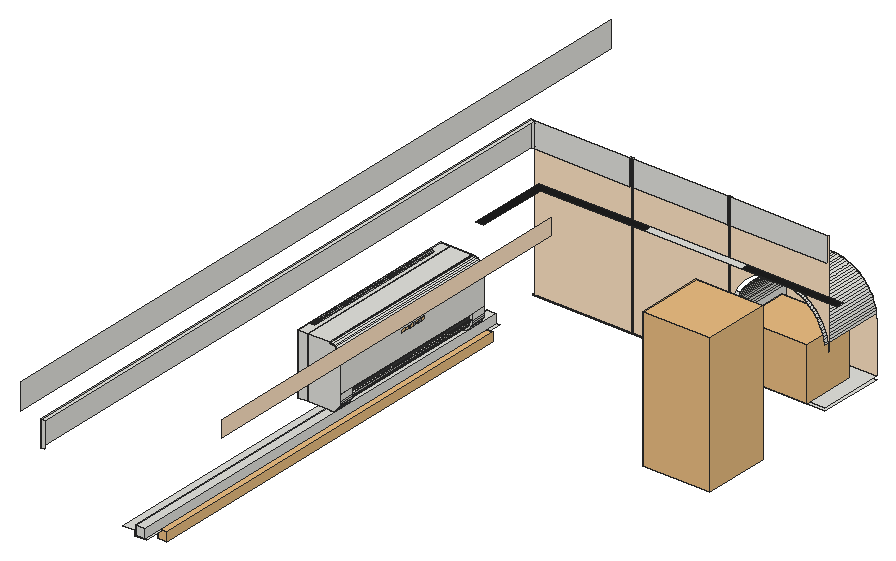
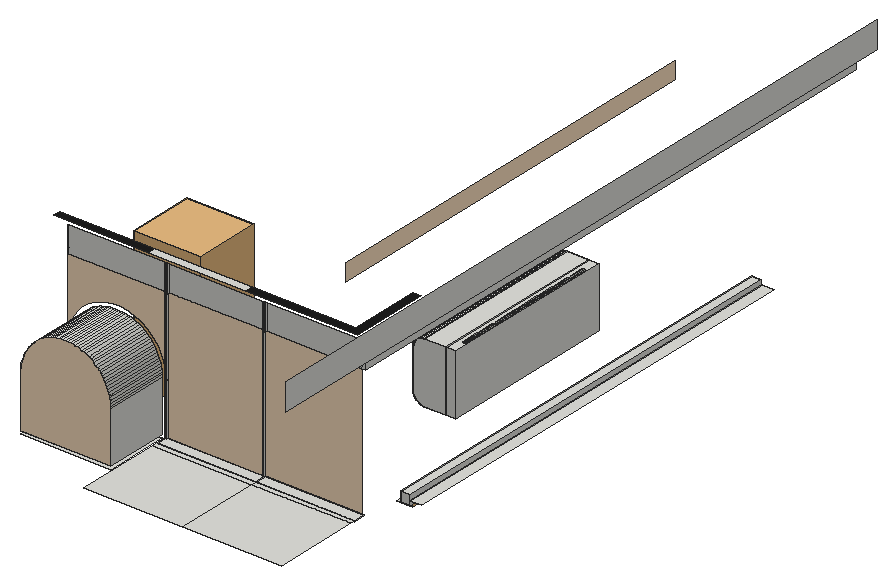
# SketchUp Ruby script. Lengths in inches.
U = 1.inch
M = Sketchup.active_model
def pt(a) = Geom::Point3d.new(a.map { |v| v * U })
def face(e, loops, mat)
  f = e.add_face(loops[0].map { |a| pt(a) })
  loops[1..].each { |l| e.add_face(l.map { |a| pt(a) }).erase! }
  f.material = f.back_material = mat if mat
  f
end
# faces: each face lists its corners as indices into pts; further lists are holes
def faces(e, pts, list, mat = nil) = list.each { |f| face(e, (f[0].is_a?(Array) ? f : [f]).map { |l| l.map { |i| pts[i] } }, mat) }
# xy, xz, yz: faces in a plane at the given z, y or x. An outline is a flat list of corners, or four numbers for a rectangle; further outlines are holes
def ring(l) = l.size == 4 ? [[l[0], l[1]], [l[2], l[1]], [l[2], l[3]], [l[0], l[3]]] : l.each_slice(2).to_a
def flat(e, list, mat, &to3) = list.each { |f| face(e, (f[0].is_a?(Array) ? f : [f]).map { |l| ring(l).map { |u, v| to3.(u, v) } }, mat) }
def xy(e, z, list, mat = nil) = flat(e, list, mat) { |x, y| [x, y, z] }
def xz(e, y, list, mat = nil) = flat(e, list, mat) { |x, z| [x, y, z] }
def yz(e, x, list, mat = nil) = flat(e, list, mat) { |y, z| [x, y, z] }
def lines(e, pts, list) = list.each { |a, b| e.add_line(pt(pts[a]), pt(pts[b])) }
# prism: a flat outline (further loops are holes) pulled along v
def prism(e, loops, v, mat = nil)
  f = face(e, loops, mat); d = Geom::Vector3d.new(v.map { |x| x * U })
  f.pushpull(f.normal.samedirection?(d) ? d.length : -d.length)
end
def box(e, o, s, mat = nil) = prism(e, [[o, [o[0] + s[0], o[1], o[2]], [o[0] + s[0], o[1] + s[1], o[2]], [o[0], o[1] + s[1], o[2]]]], [0, 0, s[2]], mat)
def at(x, y, z, deg = 0) = Geom::Transformation.translation(pt([x, y, z])) * Geom::Transformation.rotation(ORIGIN, Z_AXIS, deg.degrees)
def axes(o, x, y, z) = Geom::Transformation.new([*x, 0, *y, 0, *z, 0, *pt(o).to_a, 1])
def part(name) = M.definitions.add(name)
# library, detail: a bought-in or finely detailed component or shape, given as its bounding box
def library(name, o, s) = part(name).tap { |d| box(d.entities, o, s) }
def detail(e, o, s) = box(e.add_group.entities, o, s)
def put(e, d, t, mat = nil) = e.add_instance(d, t).tap { |i| i.material = mat if mat }
def group(e, t, mat = nil) = e.add_group.tap { |g| g.transformation = t; g.material = mat if mat }.entities
root = M.entities
M.materials.add("[0012_Bisque]").color = [255, 228, 196]
M.materials.add("[Color M08]").color = [30, 30, 30]
M.materials.add("[Color_004]").color = [142, 142, 142]
M.materials.add("[Color_007]").color = [58, 58, 58]
M.materials.add("[Color_C12]").color = [153, 91, 30]
c1 = library("Curtain rod",[-0.76,-0.76,-71.54],[3.88,3.88,152.54])
c2 = library("Group\#26",[-80.34,-149.03,-93.91],[1.18,2.79,3])
c3 = library("Group\#27",[-80.34,-139.83,-93.89],[1.18,2.84,2.98])
c4 = library("Group\#19",[-80.46,-65.36,-92.6],[1.38,3.58,3.59])
c5 = library("Group\#15",[-88.79,0.67,-41.3125],[0.99,6.14,4.87])
c6 = library("Group\#18",[-88.79,21.34,-41.3125],[0.99,6.53,4.87])
c7 = library("books",[6.19,-1.3125,-0.22],[15.35,11.9,12.07])
c8 = library("Group\#46",[0,0,0],[110.16,110.16,227.25])
xy(root,87,[[[2.71,29.49,5.62,131.05],[2.85,29.63,4.97,130.91]]])
xy(root,88.0625,[[0,29.49,2.71,131.05]])
xy(root,88.24,[[51.69,141.2,72.61,155.95]])
xy(root,88.4375,[[5.12,141.2,5.62,143.84],[5.62,141.2,27.93,143.84],[27.93,141.2,50.74,143.84],[27.56,143.84,27.93,144.02]])
xy(root,88.6875,[[5.12,141.2,27.93,143.84],[27.93,141.2,28.23,141.5],[28.23,141.2,50.44,141.2,50.44,141.5,50.74,141.5,50.74,143.84,27.93,143.84,27.93,141.5,28.23,141.5],[50.44,141.2,50.74,141.5],[5.12,143.84,27.93,145.09],
  [27.93,143.84,50.74,145.09],[5.12,145.09,27.93,164.88],[27.93,145.09,50.74,164.88]])
xy(root,88.95,[[51.69,141.2,72.61,155.95]])
xy(root,89.125,[[2.85,29.63,4.97,130.91]])
xy(root,118.75,[[39.875,130.07,62.26,131.88]])
xy(root,118.75,[[14.13,113.7,14.13,131.88,39.875,131.88,39.875,130.07,15.9375,130.07,15.9375,113.7],[62.26,130.07,84.16,131.88]],"[Color M08]")
xy(root,124.6875,[[4.82,0,5.62,141.2],[27.63,141.2,27.93,141.5],[27.93,141.2,28.23,141.5],[50.14,141.2,50.44,141.5],[50.44,141.2,50.74,141.5]])
xz(root,0,[[4.82,118.75,5.62,124.6875]])
xz(root,29.63,[[2.85,87,4.97,89.125]])
xz(root,130.91,[[2.85,87,4.97,89.125]])
xz(root,141.2,[[5.12,88.4375,5.62,88.6875],[5.62,88.4375,27.93,88.6875],[27.93,88.4375,50.74,88.6875],[4.82,118.75,5.62,124.6875],[5.62,118.75,27.63,124.6875],
  [27.93,118.75,28.23,124.6875],[28.23,118.75,50.14,124.6875],[50.44,118.75,50.74,124.6875],[50.74,118.75,73.26,124.6875]])
xz(root,141.2,[[5.62,88.6875,27.93,88.6875,27.93,124.6875,27.63,124.6875,27.63,118.75,5.62,118.75],[28.23,88.6875,50.44,88.6875,50.44,124.6875,50.14,124.6875,50.14,118.75,28.23,118.75],[50.74,100.6875,50.76,101.28,50.81,101.88,50.88,102.47,50.99,103.06,51.13,103.64,51.3,104.21,51.5,104.78,51.73,105.33,51.99,105.87,52.27,106.39,52.58,106.9,52.92,107.39,53.29,107.87,53.67,108.32,54.09,108.75,54.52,109.16,54.97,109.55,55.45,109.92,55.9375,110.25,56.45,110.57,56.97,110.85,57.51,111.11,58.0625,111.34,58.625,111.54,59.2,111.71,59.78,111.85,60.37,111.95,60.96,112.03,61.55,112.08,62.15,112.09,62.75,112.08,63.34,112.03,63.9375,111.95,64.52,111.85,65.1,111.71,65.68,111.54,66.24,111.34,66.79,111.11,67.33,110.85,67.85,110.57,68.36,110.25,68.86,109.92,69.33,109.55,69.78,109.16,70.22,108.75,70.63,108.32,71.02,107.87,71.38,107.39,71.72,106.9,72.03,106.39,72.32,105.87,72.57,105.33,72.8,104.78,73,104.21,73.17,103.64,73.31,103.06,73.42,102.47,73.5,101.88,73.54,101.28,73.56,100.6875,73.56,124.6875,73.26,124.6875,73.26,118.75,50.74,118.75]],"[0012_Bisque]")
xz(root,141.5,[[27.93,88.6875,28.23,124.6875],[50.44,88.6875,50.74,124.6875],[27.63,118.75,27.93,124.6875],[50.14,118.75,50.44,124.6875]])
xz(root,143.84,[[5.12,88.4375,27.93,88.6875],[27.93,88.4375,50.74,88.6875]])
xz(root,155.95,[[51.69,88.95,72.61,88.95,72.61,100.6875,72.59,101.23,72.55,101.78,72.48,102.32,72.38,102.86,72.25,103.39,72.1,103.92,71.91,104.43,71.7,104.94,71.47,105.43,71.21,105.92,70.92,106.38,70.61,106.83,70.28,107.27,69.92,107.68,69.55,108.08,69.15,108.46,68.73,108.8125,68.3,109.15,67.85,109.46,67.38,109.74,66.9,110,66.4,110.24,65.9,110.45,65.38,110.63,64.86,110.79,64.33,110.92,63.79,111.02,63.24,111.09,62.7,111.13,62.15,111.14,61.6,111.13,61.06,111.09,60.52,111.02,59.98,110.92,59.44,110.79,58.92,110.63,58.4,110.45,57.9,110.24,57.4,110,56.92,109.74,56.46,109.46,56,109.15,55.57,108.8125,55.15,108.46,54.76,108.08,54.38,107.68,54.02,107.27,53.69,106.83,53.38,106.38,53.1,105.92,52.83,105.43,52.6,104.94,52.39,104.43,52.21,103.92,52.05,103.39,51.92,102.86,51.82,102.32,51.75,101.78,51.71,101.23,51.69,100.6875]],"[0012_Bisque]")
yz(root,0,[[0,124.6875,170.3125,130.6875]])
yz(root,2.71,[[29.49,87,131.05,88.0625]])
yz(root,2.85,[[29.63,87,130.91,89.125]])
yz(root,4.82,[[0,118.75,141.2,124.6875]])
yz(root,4.97,[[29.63,87,130.91,89.125]])
yz(root,5.12,[[141.2,88.4375,143.84,88.6875]])
yz(root,27.63,[[141.2,118.75,141.5,124.6875]])
yz(root,27.93,[[141.2,88.4375,143.84,88.6875],[141.2,88.6875,141.5,118.75],[141.2,118.75,141.5,124.6875]])
yz(root,27.94,[[23.13,118.75,118.07,122.5625]],"[0012_Bisque]")
yz(root,28.23,[[141.2,88.6875,141.5,124.6875]])
yz(root,50.14,[[141.2,118.75,141.5,124.6875]])
yz(root,50.44,[[141.2,88.6875,141.5,100.6875],[141.2,100.6875,141.5,118.75],[141.2,118.75,141.5,124.6875]])
yz(root,50.74,[[141.2,88.4375,143.84,88.6875],[141.2,88.6875,141.5,100.6875],[141.2,100.6875,141.5,124.6875]])
yz(root,51.69,[[141.2,88.95,155.95,100.6875]])
p = [[51.71,141.2,101.23],[51.69,141.2,100.6875],[51.69,155.95,100.6875],[51.71,155.95,101.23],[51.75,141.2,101.78],[51.75,155.95,101.78],
  [51.82,141.2,102.32],[51.82,155.95,102.32],[72.55,141.2,101.78],[72.48,141.2,102.32],[72.48,155.95,102.32],[72.55,155.95,101.78],
  [51.92,141.2,102.86],[51.92,155.95,102.86],[72.38,141.2,102.86],[72.38,155.95,102.86],[52.05,141.2,103.39],[52.05,155.95,103.39],
  [72.25,141.2,103.39],[72.25,155.95,103.39],[52.21,141.2,103.92],[52.21,155.95,103.92],[72.1,141.2,103.92],[72.1,155.95,103.92],
  [52.39,141.2,104.43],[52.39,155.95,104.43],[71.91,141.2,104.43],[71.91,155.95,104.43],[52.6,141.2,104.94],[52.6,155.95,104.94],
  [71.7,141.2,104.94],[71.7,155.95,104.94],[52.83,141.2,105.43],[52.83,155.95,105.43],[71.47,141.2,105.43],[71.47,155.95,105.43],
  [53.1,141.2,105.92],[53.1,155.95,105.92],[71.21,141.2,105.92],[71.21,155.95,105.92],[53.38,141.2,106.38],[53.38,155.95,106.38],
  [70.92,141.2,106.38],[70.92,155.95,106.38],[53.69,141.2,106.83],[53.69,155.95,106.83],[70.61,141.2,106.83],[70.61,155.95,106.83],
  [54.02,141.2,107.27],[54.02,155.95,107.27],[70.28,141.2,107.27],[70.28,155.95,107.27],[54.38,141.2,107.68],[54.38,155.95,107.68],
  [69.92,141.2,107.68],[69.92,155.95,107.68],[54.76,141.2,108.08],[54.76,155.95,108.08],[69.55,141.2,108.08],[69.55,155.95,108.08],
  [55.15,141.2,108.46],[55.15,155.95,108.46],[69.15,141.2,108.46],[69.15,155.95,108.46],[55.57,141.2,108.8125],[55.57,155.95,108.8125],
  [68.73,141.2,108.8125],[68.73,155.95,108.8125],[56,141.2,109.15],[56,155.95,109.15],[68.3,141.2,109.15],[68.3,155.95,109.15],
  [56.46,141.2,109.46],[56.46,155.95,109.46],[67.85,141.2,109.46],[67.85,155.95,109.46],[56.92,141.2,109.74],[56.92,155.95,109.74],
  [67.38,141.2,109.74],[67.38,155.95,109.74],[57.4,141.2,110],[57.4,155.95,110],[66.9,141.2,110],[66.9,155.95,110],
  [57.9,141.2,110.24],[57.9,155.95,110.24],[66.4,141.2,110.24],[66.4,155.95,110.24],[58.4,141.2,110.45],[58.4,155.95,110.45],
  [65.9,141.2,110.45],[65.9,155.95,110.45],[58.92,141.2,110.63],[58.92,155.95,110.63],[65.38,141.2,110.63],[65.38,155.95,110.63],
  [59.44,141.2,110.79],[59.44,155.95,110.79],[64.86,141.2,110.79],[64.86,155.95,110.79],[59.98,141.2,110.92],[59.98,155.95,110.92],
  [64.33,141.2,110.92],[64.33,155.95,110.92],[60.52,141.2,111.02],[60.52,155.95,111.02],[63.79,141.2,111.02],[63.79,155.95,111.02],
  [61.06,141.2,111.09],[61.06,155.95,111.09],[63.24,141.2,111.09],[63.24,155.95,111.09],[61.6,141.2,111.13],[61.6,155.95,111.13],
  [62.15,141.2,111.14],[62.15,155.95,111.14],[62.7,141.2,111.13],[62.7,155.95,111.13]]
faces(root,p,[[0,1,2,3],[4,0,3,5],[6,4,5,7],[8,9,10,11],[12,6,7,13],[9,14,15,10],[16,12,13,17],[14,18,19,15],
  [20,16,17,21],[18,22,23,19],[24,20,21,25],[22,26,27,23],[28,24,25,29],[26,30,31,27],[32,28,29,33],[30,34,35,31],
  [36,32,33,37],[34,38,39,35],[40,36,37,41],[38,42,43,39],[44,40,41,45],[42,46,47,43],[48,44,45,49],[46,50,51,47],
  [52,48,49,53],[50,54,55,51],[56,52,53,57],[54,58,59,55],[60,56,57,61],[58,62,63,59],[64,60,61,65],[62,66,67,63],
  [68,64,65,69],[66,70,71,67],[72,68,69,73],[70,74,75,71],[76,72,73,77],[74,78,79,75],[80,76,77,81],[78,82,83,79],
  [84,80,81,85],[82,86,87,83],[88,84,85,89],[86,90,91,87],[92,88,89,93],[90,94,95,91],[96,92,93,97],[94,98,99,95],
  [100,96,97,101],[98,102,103,99],[104,100,101,105],[102,106,107,103],[108,104,105,109],[106,110,111,107],[112,108,109,113],[114,112,113,115],
  [116,114,115,117],[110,116,117,111]])
put(root,c1,axes([4.76,78.21,86.66],[0,0,-0.55078],[0.55078,0,0],[0,0.61526,0]))
g1 = group(root,at(5.12,94.18,110.96))
xy(g1,-13.99,[[0,-20.6,2.23,20.6]])
xy(g1,-2.49,[[0.18,-17.22,0.45,-13.11],[0.5625,-17.22,0.83,-13.11],[0.9375,-17.22,1.21,-13.11],[0.18,-12.88,0.45,-8.77],[0.5625,-12.88,0.83,-8.77],
  [0.9375,-12.88,1.21,-8.77],[0.18,-8.55,0.45,-4.44],[0.5625,-8.55,0.83,-4.44],[0.9375,-8.55,1.21,-4.44],[0.18,-4.22,0.45,-0.11],
  [0.5625,-4.22,0.83,-0.11],[0.9375,-4.22,1.21,-0.11],[0.18,0.11,0.45,4.22],[0.5625,0.11,0.83,4.22],[0.9375,0.11,1.21,4.22],
  [0.18,4.44,0.45,8.55],[0.5625,4.44,0.83,8.55],[0.9375,4.44,1.21,8.55],[0.18,8.77,0.45,12.88],[0.5625,8.77,0.83,12.88],
  [0.9375,8.77,1.21,12.88],[0.18,13.11,0.45,17.22],[0.5625,13.11,0.83,17.22],[0.9375,13.11,1.21,17.22]])
xy(g1,0,[[[0,-20.6,2.23,20.6],[0.9375,-12.88,0.9375,-8.77,1.21,-8.77,1.21,-8.55,0.9375,-8.55,0.9375,-4.44,1.21,-4.44,1.21,-12.88],[0.18,-12.88,0.18,-4.44,0.45,-4.44,0.45,-8.55,0.18,-8.55,0.18,-8.77,0.45,-8.77,0.45,-12.88],[0.5625,-17.22,0.83,-13.11],[0.18,-17.22,0.45,-13.11],[0.9375,-17.22,1.21,-13.11],[0.9375,13.11,1.21,17.22],[0.18,13.11,0.45,17.22],[0.5625,13.11,0.83,17.22],[0.5625,-8.55,0.83,-4.44],[0.18,4.44,0.45,8.55],[0.5625,4.44,0.83,8.55],[0.9375,4.44,1.21,8.55],[0.5625,-12.88,0.83,-8.77],[0.5625,-4.22,0.83,-0.11],[0.18,-4.22,0.45,-0.11],[0.9375,-4.22,1.21,-0.11],[0.18,8.77,0.45,12.88],[0.9375,8.77,1.21,12.88],[0.9375,0.11,1.21,4.22],[0.5625,0.11,0.83,4.22],[0.18,0.11,0.45,4.22],[0.5625,8.77,0.83,12.88]]])
xz(g1,-20.6,[[0,-13.99,2.23,0]])
xz(g1,-17.22,[[0.18,-2.49,0.45,0],[0.5625,-2.49,0.83,0],[0.9375,-2.49,1.21,0]])
xz(g1,-13.11,[[0.18,-2.49,0.45,0],[0.5625,-2.49,0.83,0],[0.9375,-2.49,1.21,0]])
xz(g1,-12.88,[[0.18,-2.49,0.45,0],[0.5625,-2.49,0.83,0],[0.9375,-2.49,1.21,0]])
xz(g1,-8.77,[[0.18,-2.49,0.45,0],[0.5625,-2.49,0.83,0],[0.9375,-2.49,1.21,0]])
xz(g1,-8.55,[[0.18,-2.49,0.45,0],[0.5625,-2.49,0.83,0],[0.9375,-2.49,1.21,0]])
xz(g1,-4.44,[[0.18,-2.49,0.45,0],[0.5625,-2.49,0.83,0],[0.9375,-2.49,1.21,0]])
xz(g1,-4.22,[[0.18,-2.49,0.45,0],[0.5625,-2.49,0.83,0],[0.9375,-2.49,1.21,0]])
xz(g1,-0.11,[[0.18,-2.49,0.45,0],[0.5625,-2.49,0.83,0],[0.9375,-2.49,1.21,0]])
xz(g1,0.11,[[0.18,-2.49,0.45,0],[0.5625,-2.49,0.83,0],[0.9375,-2.49,1.21,0]])
xz(g1,4.22,[[0.18,-2.49,0.45,0],[0.5625,-2.49,0.83,0],[0.9375,-2.49,1.21,0]])
xz(g1,4.44,[[0.18,-2.49,0.45,0],[0.5625,-2.49,0.83,0],[0.9375,-2.49,1.21,0]])
xz(g1,8.55,[[0.18,-2.49,0.45,0],[0.5625,-2.49,0.83,0],[0.9375,-2.49,1.21,0]])
xz(g1,8.77,[[0.18,-2.49,0.45,0],[0.5625,-2.49,0.83,0],[0.9375,-2.49,1.21,0]])
xz(g1,12.88,[[0.18,-2.49,0.45,0],[0.5625,-2.49,0.83,0],[0.9375,-2.49,1.21,0]])
xz(g1,13.11,[[0.18,-2.49,0.45,0],[0.5625,-2.49,0.83,0],[0.9375,-2.49,1.21,0]])
xz(g1,17.22,[[0.18,-2.49,0.45,0],[0.5625,-2.49,0.83,0],[0.9375,-2.49,1.21,0]])
xz(g1,20.6,[[0,-13.99,2.23,0]])
yz(g1,0,[[-20.6,-13.99,20.6,0]])
yz(g1,0.18,[[-17.22,-2.49,-13.11,0],[-12.88,-2.49,-8.77,0],[-8.55,-2.49,-4.44,0],[-4.22,-2.49,-0.11,0],[0.11,-2.49,4.22,0],
  [4.44,-2.49,8.55,0],[8.77,-2.49,12.88,0],[13.11,-2.49,17.22,0]])
yz(g1,0.45,[[-17.22,-2.49,-13.11,0],[-12.88,-2.49,-8.77,0],[-8.55,-2.49,-4.44,0],[-4.22,-2.49,-0.11,0],[0.11,-2.49,4.22,0],
  [4.44,-2.49,8.55,0],[8.77,-2.49,12.88,0],[13.11,-2.49,17.22,0]])
yz(g1,0.5625,[[-17.22,-2.49,-13.11,0],[-12.88,-2.49,-8.77,0],[-8.55,-2.49,-4.44,0],[-4.22,-2.49,-0.11,0],[0.11,-2.49,4.22,0],
  [4.44,-2.49,8.55,0],[8.77,-2.49,12.88,0],[13.11,-2.49,17.22,0]])
yz(g1,0.83,[[-17.22,-2.49,-13.11,0],[-12.88,-2.49,-8.77,0],[-8.55,-2.49,-4.44,0],[-4.22,-2.49,-0.11,0],[0.11,-2.49,4.22,0],
  [4.44,-2.49,8.55,0],[8.77,-2.49,12.88,0],[13.11,-2.49,17.22,0]])
yz(g1,0.9375,[[-17.22,-2.49,-13.11,0],[-12.88,-2.49,-8.77,0],[-8.55,-2.49,-4.44,0],[-4.22,-2.49,-0.11,0],[0.11,-2.49,4.22,0],
  [4.44,-2.49,8.55,0],[8.77,-2.49,12.88,0],[13.11,-2.49,17.22,0]])
yz(g1,1.21,[[-17.22,-2.49,-13.11,0],[-12.88,-2.49,-8.77,0],[-8.55,-2.49,-4.44,0],[-4.22,-2.49,-0.11,0],[0.11,-2.49,4.22,0],
  [4.44,-2.49,8.55,0],[8.77,-2.49,12.88,0],[13.11,-2.49,17.22,0]])
yz(g1,2.23,[[-20.6,-13.99,20.6,0]])
g2 = group(root,at(5.12,94.18,110.96))
xy(g2,-13.99,[[2.23,-20.6,7.28,-17.4375],[2.23,17.4375,7.28,20.6]])
xy(g2,-10.88,[[2.23,-17.4375,9.07,17.4375]])
xy(g2,-10.66,[[8.9375,-3.83,9.07,3.83]])
xy(g2,-9.96,[[8.9375,-3.83,9.07,3.83]])
xy(g2,-9.84,[[9.83,-20.6,9.97,-17.4375],[9.07,-17.4375,9.83,17.4375],[9.83,17.4375,9.97,20.6]])
xy(g2,0,[[2.23,-20.6,7.28,20.6]])
xz(g2,-20.6,[[2.23,-13.99,7.28,-13.99,7.7,-13.96,8.11,-13.86,8.5,-13.7,8.86,-13.48,9.18,-13.2,9.45,-12.88,9.67,-12.52,9.84,-12.14,9.93,-11.73,9.97,-11.31,9.97,-9.84,9.83,-9.84,9.83,-2.68,9.8,-2.28,9.71,-1.89,9.55,-1.53,9.35,-1.18,9.09,-0.88,8.78,-0.62,8.44,-0.41,8.07,-0.26,7.68,-0.17,7.28,-0.13,7.28,0,2.23,0]])
xz(g2,-17.4375,[[2.23,-13.99,2.23,-10.88,9.07,-10.88,9.07,-9.84,9.97,-9.84,9.97,-11.31,9.93,-11.73,9.84,-12.14,9.67,-12.52,9.45,-12.88,9.18,-13.2,8.86,-13.48,8.5,-13.7,8.11,-13.86,7.7,-13.96,7.28,-13.99]])
xz(g2,-3.83,[[8.9375,-10.66,9.07,-9.96]])
xz(g2,3.83,[[8.9375,-10.66,9.07,-9.96]])
xz(g2,17.4375,[[2.23,-13.99,7.28,-13.99,7.7,-13.96,8.11,-13.86,8.5,-13.7,8.86,-13.48,9.18,-13.2,9.45,-12.88,9.67,-12.52,9.84,-12.14,9.93,-11.73,9.97,-11.31,9.97,-9.84,9.07,-9.84,9.07,-10.88,2.23,-10.88]])
xz(g2,20.6,[[2.23,-13.99,2.23,0,7.28,0,7.28,-0.13,7.68,-0.17,8.07,-0.26,8.44,-0.41,8.78,-0.62,9.09,-0.88,9.35,-1.18,9.55,-1.53,9.71,-1.89,9.8,-2.28,9.83,-2.68,9.83,-9.84,9.97,-9.84,9.97,-11.31,9.93,-11.73,9.84,-12.14,9.67,-12.52,9.45,-12.88,9.18,-13.2,8.86,-13.48,8.5,-13.7,8.11,-13.86,7.7,-13.96,7.28,-13.99]])
yz(g2,2.23,[[-20.6,-13.99,-20.6,0,20.6,0,20.6,-13.99,17.4375,-13.99,17.4375,-10.88,-17.4375,-10.88,-17.4375,-13.99]])
yz(g2,7.28,[[-20.6,-0.13,20.6,0]])
yz(g2,8.9375,[[-3.83,-10.66,3.83,-9.96]],"[Color_007]")
yz(g2,9.07,[[[-17.4375,-10.88,17.4375,-9.84],[-3.83,-10.66,3.83,-9.96]]])
yz(g2,9.83,[[-20.6,-9.84,20.6,-2.68]])
yz(g2,9.97,[[-20.6,-11.31,-17.4375,-9.84],[17.4375,-11.31,20.6,-9.84]])
p = [[7.28,-20.6,-13.99],[7.28,-17.4375,-13.99],[7.7,-17.4375,-13.96],[7.7,-20.6,-13.96],[8.11,-17.4375,-13.86],[8.11,-20.6,-13.86],
  [7.28,17.4375,-13.99],[7.28,20.6,-13.99],[7.7,20.6,-13.96],[7.7,17.4375,-13.96],[8.11,20.6,-13.86],[8.11,17.4375,-13.86],
  [8.5,-17.4375,-13.7],[8.5,-20.6,-13.7],[8.5,17.4375,-13.7],[8.5,20.6,-13.7],[8.86,-17.4375,-13.48],[8.86,-20.6,-13.48],
  [8.86,20.6,-13.48],[8.86,17.4375,-13.48],[9.18,-17.4375,-13.2],[9.18,-20.6,-13.2],[9.18,20.6,-13.2],[9.18,17.4375,-13.2],
  [9.45,-17.4375,-12.88],[9.45,-20.6,-12.88],[9.45,20.6,-12.88],[9.45,17.4375,-12.88],[9.67,-17.4375,-12.52],[9.67,-20.6,-12.52],
  [9.67,20.6,-12.52],[9.67,17.4375,-12.52],[9.84,-17.4375,-12.14],[9.84,-20.6,-12.14],[9.84,17.4375,-12.14],[9.84,20.6,-12.14],
  [9.93,-17.4375,-11.73],[9.93,-20.6,-11.73],[9.93,20.6,-11.73],[9.93,17.4375,-11.73],[9.97,-17.4375,-11.31],[9.97,-20.6,-11.31],
  [9.97,20.6,-11.31],[9.97,17.4375,-11.31],[9.83,-20.6,-2.68],[9.83,20.6,-2.68],[9.8,20.6,-2.28],[9.8,-20.6,-2.28],
  [9.71,20.6,-1.89],[9.71,-20.6,-1.89],[9.55,-20.6,-1.53],[9.55,20.6,-1.53],[9.35,20.6,-1.18],[9.35,-20.6,-1.18],
  [9.09,20.6,-0.88],[9.09,-20.6,-0.88],[8.78,20.6,-0.62],[8.78,-20.6,-0.62],[8.44,20.6,-0.41],[8.44,-20.6,-0.41],
  [8.07,-20.6,-0.26],[8.07,20.6,-0.26],[7.68,20.6,-0.17],[7.68,-20.6,-0.17],[7.28,20.6,-0.13],[7.28,-20.6,-0.13]]
faces(g2,p,[[0,1,2,3],[4,5,3,2],[6,7,8,9],[10,11,9,8],[4,12,13,5],[14,11,10,15],[13,12,16,17],[14,15,18,19],
  [20,21,17,16],[22,23,19,18],[21,20,24,25],[23,22,26,27],[28,29,25,24],[30,31,27,26],[28,32,33,29],[34,31,30,35],
  [33,32,36,37],[34,35,38,39],[40,41,37,36],[42,43,39,38],[44,45,46,47],[48,49,47,46],[50,49,48,51],[50,51,52,53],
  [54,55,53,52],[55,54,56,57],[58,59,57,56],[60,59,58,61],[60,61,62,63],[64,65,63,62]])
g3 = group(root,at(5.12,94.18,110.96))
xy(g3,-13.59,[[4.74,-17.4375,7.2,17.4375]])
xy(g3,-11.45,[[9.03,-17.4375,9.35,-5.4375],[9.03,-5.17,9.35,9.72],[9.03,9.99,9.35,17.4375]])
xy(g3,-10.88,[[4.74,-17.4375,9.03,-17.4375,9.03,-5.4375,9.35,-5.4375,9.35,-5.17,9.03,-5.17,9.03,9.72,9.35,9.72,9.35,9.99,9.03,9.99,9.03,17.4375,4.74,17.4375]])
xz(g3,-17.4375,[[4.74,-13.59,7.2,-13.59,7.54,-13.5625,7.87,-13.49,8.18,-13.36,8.46,-13.18,8.72,-12.96,8.9375,-12.71,9.11,-12.42,9.24,-12.11,9.32,-11.78,9.35,-11.49,9.35,-11.45,9.03,-11.45,9.03,-10.88,4.74,-10.88]])
xz(g3,-5.4375,[[9.03,-11.45,9.35,-10.88]])
xz(g3,-5.17,[[9.03,-11.45,9.35,-10.88]])
xz(g3,9.72,[[9.03,-11.45,9.35,-10.88]])
xz(g3,9.99,[[9.03,-11.45,9.35,-10.88]])
xz(g3,17.4375,[[4.74,-13.59,4.74,-10.88,9.03,-10.88,9.03,-11.45,9.35,-11.45,9.35,-11.49,9.32,-11.78,9.24,-12.11,9.11,-12.42,8.9375,-12.71,8.72,-12.96,8.46,-13.18,8.18,-13.36,7.87,-13.49,7.54,-13.5625,7.2,-13.59]])
yz(g3,4.74,[[-17.4375,-13.59,17.4375,-10.88]])
yz(g3,9.03,[[-17.4375,-11.45,-5.4375,-10.88],[-5.17,-11.45,9.72,-10.88],[9.99,-11.45,17.4375,-10.88]],"[Color_007]")
yz(g3,9.35,[[-5.4375,-11.45,-5.17,-10.88],[9.72,-11.45,9.99,-10.88]])
yz(g3,9.35,[[-17.4375,-11.49,17.4375,-11.45]],"[Color_C12]")
p = [[7.2,-17.4375,-13.59],[7.2,17.4375,-13.59],[7.54,17.4375,-13.5625],[7.54,-17.4375,-13.5625],[7.87,17.4375,-13.49],[7.87,-17.4375,-13.49],
  [8.18,-17.4375,-13.36],[8.18,17.4375,-13.36],[8.46,17.4375,-13.18],[8.46,-17.4375,-13.18],[8.72,17.4375,-12.96],[8.72,-17.4375,-12.96],
  [8.9375,17.4375,-12.71],[8.9375,-17.4375,-12.71],[9.11,17.4375,-12.42],[9.11,-17.4375,-12.42],[9.24,-17.4375,-12.11],[9.24,17.4375,-12.11],
  [9.32,17.4375,-11.78],[9.32,-17.4375,-11.78],[9.35,17.4375,-11.49],[9.35,9.99,-11.49],[9.35,9.72,-11.49],[9.35,-5.17,-11.49],
  [9.35,-5.4375,-11.49],[9.35,-17.4375,-11.49]]
faces(g3,p,[[0,1,2,3],[4,5,3,2],[6,5,4,7],[6,7,8,9],[10,11,9,8],[11,10,12,13],[14,15,13,12],[16,15,14,17],
  [16,17,18,19],[18,20,21,22,23,24,25,19]])
g4 = group(root,at(5.12,94.18,110.96))
prism(g4,[[[9.97,-20.58,-9.84],[9.97,-20.58,-2.68],[9.93,-20.58,-2.26],[9.84,-20.58,-1.85],[9.67,-20.58,-1.46],[9.45,-20.58,-1.11],[9.18,-20.58,-0.79],[8.86,-20.58,-0.51],[8.5,-20.58,-0.29],[8.11,-20.58,-0.13],[7.7,-20.58,-0.03],[7.28,-20.58,0],[7.28,-20.58,-0.13],[7.68,-20.58,-0.17],[8.07,-20.58,-0.26],[8.44,-20.58,-0.41],[8.78,-20.58,-0.62],[9.09,-20.58,-0.88],[9.35,-20.58,-1.18],[9.55,-20.58,-1.53],[9.71,-20.58,-1.89],[9.8,-20.58,-2.28],[9.83,-20.58,-2.68],[9.83,-20.58,-9.84]]],[0,41.16,0])
put(root,c2,axes([5.2,94.18,110.96],[-0.11352,0,0],[0,-0.11352,0],[0,0,0.11352]))
g5 = group(root,at(5.2,94.18,110.96))
detail(g5,[8.99,16.95,-10.66],[0.13,0.08,0.08])
g6 = group(root,at(5.2,94.18,110.96))
detail(g6,[8.99,15.9,-10.66],[0.13,0.28,0.45])
put(root,c3,axes([5.2,94.18,110.96],[-0.11352,0,0],[0,-0.11352,0],[0,0,0.11352]))
g7 = group(root,at(5.2,94.18,110.96),"[Color_004]")
prism(g7,[[[9.12,16.55,-10.32],[9.12,16.43,-10.55],[9.12,16.39,-10.32],[9.12,16.31,-10.32],[9.12,16.38,-10.65],[9.12,16.46,-10.65],[9.12,16.64,-10.32]]],[-0.13,0,0],"[Color_004]")
g8 = group(root,at(5.2,94.18,110.96))
prism(g8,[[[9.12,16.24,-10.65],[9.12,16.3,-10.32],[9.12,16.23,-10.32],[9.12,16.17,-10.65]]],[-0.13,0,0],"[Color_004]")
g9 = group(root,at(5.2,94.18,110.96))
prism(g9,[[[9.12,17.02,-10.21],[9.12,16.97,-10.54],[9.12,17.05,-10.54],[9.12,17.1,-10.21]]],[-0.13,0,0],"[Color_004]")
g10 = group(root,at(5.2,94.18,110.96))
detail(g10,[8.99,16.24,-10.29],[0.13,0.08,0.08])
put(root,c4,axes([5.22,94.18,110.96],[-0.11352,0,0],[0,-0.11352,0],[0,0,0.11352]))
g11 = group(root,at(5.12,94.18,110.96))
detail(g11,[9.97,-2.34,-4.69],[0.11,0.74,0.55])
g12 = group(root,at(5.12,94.18,110.96),"[Color_004]")
prism(g12,[[[9.97,1.58,-4.69],[9.97,1.4,-4.69],[9.97,1.54,-4.14],[9.97,1.77,-4.14],[9.97,1.9,-4.51],[9.97,2.02,-4.14],[9.97,2.25,-4.14],[9.97,2.39,-4.69],[9.97,2.21,-4.69],[9.97,2.11,-4.32],[9.97,2,-4.69],[9.97,1.8,-4.69],[9.97,1.68,-4.3]]],[0.11,0,0],"[Color_004]")
put(root,c5,axes([5.12,94.18,110.96],[-0.11352,0,0],[0,-0.11352,0],[0,0,0.11352]))
g13 = group(root,at(5.12,94.18,110.96))
detail(g13,[9.97,2.43,-4.69],[0.11,0.71,0.55])
g14 = group(root,at(5.12,94.18,110.96))
prism(g14,[[[9.97,-0.02,-4.27],[9.97,-0.02,-4.14],[9.97,0.59,-4.14],[9.97,0.59,-4.27],[9.97,0.39,-4.27],[9.97,0.39,-4.69],[9.97,0.1875,-4.69],[9.97,0.1875,-4.27]]],[0.11,0,0],"[Color_004]")
g15 = group(root,at(5.12,94.18,110.96))
detail(g15,[9.97,0.65,-4.69],[0.11,0.7,0.55])
g16 = group(root,at(5.12,94.18,110.96))
prism(g16,[[[9.97,0.9,-4.48],[9.97,0.84,-4.35],[9.97,1.26,-4.35],[9.97,1.35,-4.48]]],[0.11,0,0],"[Color_004]")
g17 = group(root,at(5.12,94.18,110.96))
prism(g17,[[[9.97,-1.43,-4.69],[9.97,-1.63,-4.69],[9.97,-1.33,-4.17],[9.97,-1.32,-4.16],[9.97,-1.31,-4.15],[9.97,-1.3,-4.14],[9.97,-1.29,-4.14],[9.97,-1.28,-4.14],[9.97,-1.14,-4.14],[9.97,-1.13,-4.14],[9.97,-1.12,-4.14],[9.97,-1.11,-4.15],[9.97,-1.1,-4.16],[9.97,-1.09,-4.17],[9.97,-0.79,-4.69],[9.97,-0.99,-4.69],[9.97,-1.06,-4.57],[9.97,-1.36,-4.57]],[[9.97,-1.31,-4.48],[9.97,-1.11,-4.48],[9.97,-1.21,-4.3125]]],[0.11,0,0],"[Color_004]")
put(root,c6,axes([5.12,94.18,110.96],[-0.11352,0,0],[0,-0.11352,0],[0,0,0.11352]))
put(root,c7,at(48,141.2,89.46))
put(root,c8,axes([56.07,109.31,85.03],[0.14,0,0],[0,0.14,0],[0,0,0.14]))
